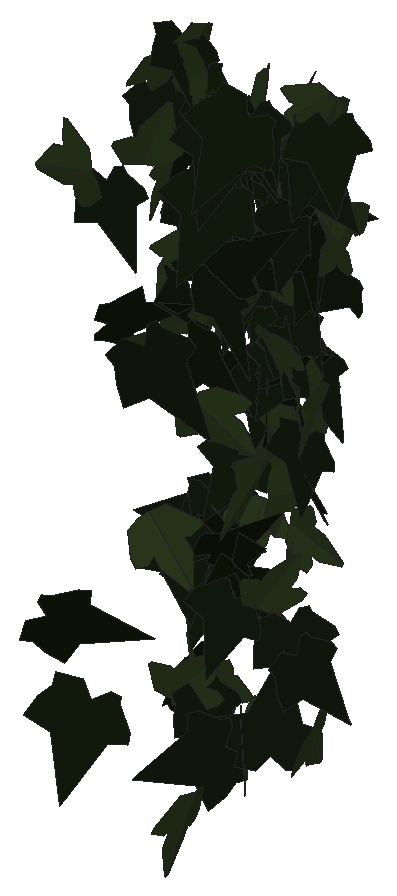
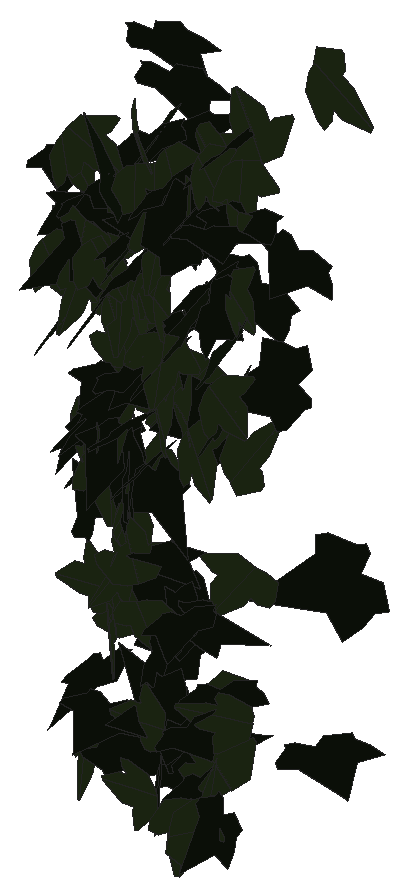
# SketchUp Ruby script. Lengths in inches.
U = 1.inch
M = Sketchup.active_model
def pt(a) = Geom::Point3d.new(a.map { |v| v * U })
def face(e, loops, mat)
  f = e.add_face(loops[0].map { |a| pt(a) })
  loops[1..].each { |l| e.add_face(l.map { |a| pt(a) }).erase! }
  f.material = f.back_material = mat if mat
  f
end
# faces: each face lists its corners as indices into pts; further lists are holes
def faces(e, pts, list, mat = nil) = list.each { |f| face(e, (f[0].is_a?(Array) ? f : [f]).map { |l| l.map { |i| pts[i] } }, mat) }
# xy, xz, yz: faces in a plane at the given z, y or x. An outline is a flat list of corners, or four numbers for a rectangle; further outlines are holes
def ring(l) = l.size == 4 ? [[l[0], l[1]], [l[2], l[1]], [l[2], l[3]], [l[0], l[3]]] : l.each_slice(2).to_a
def flat(e, list, mat, &to3) = list.each { |f| face(e, (f[0].is_a?(Array) ? f : [f]).map { |l| ring(l).map { |u, v| to3.(u, v) } }, mat) }
def xy(e, z, list, mat = nil) = flat(e, list, mat) { |x, y| [x, y, z] }
def xz(e, y, list, mat = nil) = flat(e, list, mat) { |x, z| [x, y, z] }
def yz(e, x, list, mat = nil) = flat(e, list, mat) { |y, z| [x, y, z] }
def lines(e, pts, list) = list.each { |a, b| e.add_line(pt(pts[a]), pt(pts[b])) }
# prism: a flat outline (further loops are holes) pulled along v
def prism(e, loops, v, mat = nil)
  f = face(e, loops, mat); d = Geom::Vector3d.new(v.map { |x| x * U })
  f.pushpull(f.normal.samedirection?(d) ? d.length : -d.length)
end
def box(e, o, s, mat = nil) = prism(e, [[o, [o[0] + s[0], o[1], o[2]], [o[0] + s[0], o[1] + s[1], o[2]], [o[0], o[1] + s[1], o[2]]]], [0, 0, s[2]], mat)
def at(x, y, z, deg = 0) = Geom::Transformation.translation(pt([x, y, z])) * Geom::Transformation.rotation(ORIGIN, Z_AXIS, deg.degrees)
def axes(o, x, y, z) = Geom::Transformation.new([*x, 0, *y, 0, *z, 0, *pt(o).to_a, 1])
def part(name) = M.definitions.add(name)
# library, detail: a bought-in or finely detailed component or shape, given as its bounding box
def library(name, o, s) = part(name).tap { |d| box(d.entities, o, s) }
def detail(e, o, s) = box(e.add_group.entities, o, s)
def put(e, d, t, mat = nil) = e.add_instance(d, t).tap { |i| i.material = mat if mat }
def group(e, t, mat = nil) = e.add_group.tap { |g| g.transformation = t; g.material = mat if mat }.entities
root = M.entities
M.materials.add("efeu1").color = [18, 25, 13]
M.materials.add("efeu2").color = [43, 57, 29]
c1 = part("ivyleaf_10")
p = [[0,0.5,-0.03],[-0.0625,2.02,-0.43],[-0.19,2.01,-0.46],[-0.54,1.05,-0.29],[-0.52,0.625,-0.18],[-0.83,0.76,-0.28],
  [-1.16,0.64,-0.33],[-1.15,0.33,-0.24],[-0.77,-0.39,0.02],[-0.3,-0.51,0.16],[0.04,-0.48,0.23],[-0.02,2.01,-0.4375],
  [-0.06,2.01,-0.43],[0.04,-0.49,0.23],[0.67,-0.49,0.14],[1.38,0.36,-0.2],[1.375,0.51,-0.24],[0.81,0.65,-0.19],
  [0.62,0.59,-0.15],[0.6,1.09,-0.28],[0.5,1.23,-0.31]]
faces(c1.entities,p,[[0,1,2,3,4,5,6,7,8,9,10],[11,12,0,13,14,15,16,17,18,19,20]],"efeu2")
c2 = part("ivyleaf_9")
p = [[1.54,2.16,1.25],[1.36,2.04,1.19],[-0.21,0.99,0.68],[-0.71,1.11,0.82],[-0.85,0.86,0.67],[-0.8,0.17,0.21],
  [-0.9,-0.01,0.1],[-0.67,-0.16,-0.02],[-0.08,-0.08,-0.05],[-0.03,-0.6,-0.4],[0.65,-0.88,-0.66],[0.83,-0.6,-0.49],
  [1.29,-0.42,-0.43],[1.8125,-0.07,-0.26],[1.21,0.44,0.15]]
faces(c2.entities,p,[[0,1,2,3,4,5,6,7,8,9,10,11,12,13,14]],"efeu1")
put(root,c1,axes([519.01,126.77,205.03],[-0.31987,0.03576,1.02162],[-1.02187,-0.04001,-0.31855],[0.02752,-1.06978,0.04607]))
put(root,c1,axes([521.88,127.9,184.67],[0.16584,-1.03656,0.26292],[0.06825,-0.25526,-1.04942],[1.06721,0.1774,0.02625]))
put(root,c2,axes([517.63,127,189.8],[0.13093,0.34043,-0.9819],[0.41581,0.88983,0.36395],[0.95243,-0.43528,-0.02391]))
put(root,c2,axes([520.05,128.35,198.8],[-0.14877,-0.30864,-1.04293],[0.82718,0.65139,-0.31076],[0.70622,-0.82797,0.14429]))
put(root,c2,axes([517.01,129.52,185.63],[-0.63548,-0.79383,-0.19057],[0.11492,0.15212,-1.01684],[0.80825,-0.64577,-0.00526]))
put(root,c2,axes([521.53,129.91,203.75],[-0.52245,-0.87618,0.11869],[-0.0636,-0.10026,-1.02012],[0.8819,-0.5263,-0.00326]))
put(root,c2,axes([522.52,129.74,206.55],[-0.92389,-0.45387,-0.15194],[0.13673,0.06627,-1.02935],[0.45868,-0.93395,0.0008]))
put(root,c2,axes([521.48,129.72,200.92],[0.47858,-0.90282,-0.01651],[-0.00454,0.01629,-1.02182],[0.90296,0.47859,0.00362]))
put(root,c2,axes([521.63,130.19,205.73],[-0.82447,-0.51633,-0.33937],[0.29967,0.16074,-0.97257],[0.54035,-0.87698,0.02155]))
put(root,c1,axes([518.93,129.84,204.1875],[-0.46617,-0.77023,0.19402],[0.10362,0.16408,0.90031],[-0.7875,0.47753,0.00361]))
put(root,c2,axes([521.22,129.75,200.97],[0.02313,-0.08298,1.0143],[1.00331,0.17177,-0.00883],[-0.17043,0.99992,0.08569]))
put(root,c2,axes([520.66,131,184.8],[-0.0399,-0.47857,-0.87325],[0.1005,-0.87143,0.47297],[-0.99071,-0.06912,0.08315]))
put(root,c1,axes([520.78,130.08,196.41],[-0.75552,-0.27252,-0.60479],[0.55997,0.22939,-0.80291],[0.35562,-0.94019,-0.0206]))
put(root,c1,axes([521.46,131.29,193.6],[0.19021,-0.33456,0.88892],[0.38201,-0.80307,-0.38399],[0.86959,0.42596,-0.02575]))
put(root,c2,axes([516.74,130.71,202],[-0.38724,-0.30191,-0.75298],[0.62895,0.41527,-0.48996],[0.51239,-0.7379,0.03234]))
put(root,c1,axes([518.38,130.89,191.24],[0.67878,0.4004,0.57075],[0.49981,0.27589,-0.78796],[-0.48606,0.84284,-0.01322]))
put(root,c2,axes([516.99,130.57,197.64],[0.43513,0.28551,0.7271],[0.5825,0.43596,-0.51978],[-0.52047,0.72661,0.02615]))
put(root,c1,axes([521.19,131.46,199.2],[0.23654,-0.91313,-0.24005],[0.05873,-0.23276,0.94327],[-0.94232,-0.24372,-0.00147]))
put(root,c2,axes([520.61,132.1,205],[0.46524,-0.7141,-0.10338],[-0.04716,0.09265,-0.85221],[0.72,0.46749,0.01098]))
put(root,c2,axes([519.81,132.57,188.63],[-0.23336,-0.81643,0.19969],[-0.03743,-0.19695,-0.84894],[0.83966,-0.23568,0.01765]))
put(root,c2,axes([520.83,132.21,204.93],[0.01502,-0.75793,-0.37824],[0.04097,0.3785,-0.75684],[0.84608,-0.00487,0.04336]))
put(root,c1,axes([518.375,132.03,185.42],[-0.64156,-0.45455,0.48942],[0.39772,0.28524,0.78626],[-0.53663,0.75483,-0.00239]))
put(root,c2,axes([518.7,132.1,196.88],[-0.01661,-0.01432,-0.94426],[0.8476,0.41621,-0.02122],[0.41642,-0.84775,0.00553]))
put(root,c2,axes([520.18,132.58,184.54],[0.08773,-0.14272,-0.8229],[0.78761,-0.26113,0.12926],[-0.27785,-0.78528,0.10657]))
put(root,c2,axes([521,132.64,200.29],[0.40363,-0.90769,0.0306],[-0.01224,0.02805,0.99339],[-0.90813,-0.40382,0.00021]))
put(root,c1,axes([520,132.31,204.36],[0.00735,-0.83915,0.07771],[0.00116,-0.07771,-0.83918],[0.84274,0.00742,0.00048]))
put(root,c1,axes([517.14,132.84,195.9375],[-0.13269,-0.35305,-0.84263],[-0.27619,-0.79613,0.37706],[-0.87086,0.30628,0.00881]))
put(root,c1,axes([521.41,132.15,189.47],[-0.34614,-0.67975,0.38224],[0.19274,0.33066,0.76256],[-0.75566,0.39571,0.01941]))
put(root,c2,axes([521.65,132.01,184.62],[-0.81437,-0.19451,0.51813],[0.5031,0.12392,0.83727],[-0.23061,0.95723,-0.00311]))
put(root,c2,axes([521.72,132.9375,201.58],[-0.10971,-0.79954,0.25874],[0.05016,-0.2667,-0.80287],[0.83887,-0.08862,0.08185]))
put(root,c2,axes([519.9,132.85,199.24],[-0.2366,-0.78834,0.02024],[-0.00511,-0.0196,-0.82308],[0.78858,-0.23665,0.00074]))
put(root,c2,axes([518.86,132.4375,185.26],[0.14733,-0.72504,-0.4325],[-0.07048,0.42694,-0.73973],[0.8413,0.16274,0.01377]))
put(root,c2,axes([518.31,132.75,201.31],[0.08268,-0.80664,-0.15809],[0.00292,0.15917,-0.81065],[0.82198,0.08057,0.01878]))
put(root,c2,axes([522.13,132.98,194.54],[-0.01234,-0.81617,0.10867],[0.0207,-0.10895,-0.81596],[0.82311,-0.0095,0.02215]))
put(root,c1,axes([518.64,132.41,205.61],[0.45137,-0.30497,-0.6524],[-0.50379,0.41648,-0.54324],[0.51462,0.6752,0.04041]))
put(root,c2,axes([519.3125,132.38,190.15],[0.50725,0.73315,-0.17413],[0.09541,0.14573,0.89151],[0.74748,-0.51613,0.00437]))
put(root,c2,axes([522.39,132.41,187.72],[0.27416,-0.5404,-0.6401],[-0.14338,0.6333,-0.59607],[0.82535,0.28952,0.10908]))
put(root,c2,axes([519.13,132.96,190.14],[0.10308,-0.20205,0.79884],[0.59706,-0.53653,-0.21274],[0.56789,0.60076,0.07867]))
put(root,c2,axes([521.96,133.23,192.98],[0.16199,-0.37225,0.7742],[0.36744,-0.68211,-0.40485],[0.77649,0.40044,0.03006]))
put(root,c1,axes([522.8,132.48,185.32],[0.08208,-0.72855,-0.48451],[-0.04713,0.48225,-0.73314],[0.87368,0.09446,0.00597]))
put(root,c2,axes([519.36,132.95,203.16],[-0.27153,-0.22066,-0.81665],[0.78986,0.24095,-0.32773],[0.30287,-0.82619,0.12253]))
put(root,c2,axes([518.49,133.35,203.74],[0.05889,-0.76881,0.33445],[0.05568,-0.33094,-0.77057],[0.83656,0.07615,0.02775]))
put(root,c1,axes([520.43,133.19,205.56],[0.5417,-0.4128,0.53936],[0.42723,-0.32923,-0.68106],[0.52801,0.68989,-0.00228]))
put(root,c2,axes([518.63,133.04,190.7],[-0.30926,-0.24955,-0.7248],[-0.564,-0.45524,0.39738],[-0.51915,0.64322,0.00005]))
put(root,c1,axes([516.95,133.27,201.7],[0.26054,-0.68935,0.42023],[0.17032,-0.3847,-0.73667],[0.78917,0.31061,0.02025]))
put(root,c2,axes([522.03,133.27,201.16],[-0.28354,-0.16781,-0.80142],[0.81859,-0.03867,-0.28152],[0.01876,-0.84922,0.17118]))
put(root,c1,axes([522.34,133.41,195.8],[0.2956,-0.62662,0.51847],[0.22332,-0.46791,-0.69284],[0.78205,0.37047,0.00187]))
put(root,c2,axes([517.5,133.22,205.96],[0.1942,-0.86612,-0.10074],[-0.00267,0.10262,-0.88741],[0.87196,0.19322,0.01972]))
put(root,c1,axes([520.3,133.12,184.66],[-0.16319,0.02788,-0.82667],[0.76294,-0.32042,-0.16141],[-0.31952,-0.77933,0.03679]))
put(root,c2,axes([517.41,133.59,197.23],[0.51341,-0.572,-0.38851],[0.24292,-0.30384,0.76836],[-0.64739,-0.56764,-0.01979]))
put(root,c1,axes([516.99,132.89,205.28],[-0.29687,-0.7823,-0.20791],[0.04851,0.20386,-0.83633],[0.808,-0.29967,-0.02617]))
put(root,c2,axes([519.0625,132.92,200.11],[0.25475,-0.64378,-0.46681],[0.03017,0.49765,-0.66985],[0.79464,0.18749,0.17509]))
put(root,c1,axes([520.125,133.49,200.42],[0.36037,-0.63469,0.58028],[0.34551,-0.4693,-0.72788],[0.78752,0.49634,0.0538]))
put(root,c1,axes([521.07,132.91,197.37],[-0.83559,0.17919,-0.02298],[0.02243,-0.00499,-0.85458],[-0.17926,-0.83589,0.00018]))
put(root,c2,axes([519.41,133.35,204.24],[0.06442,-0.83473,-0.10782],[-0.02085,0.10651,-0.83712],[0.84141,0.06655,-0.01249]))
put(root,c1,axes([520.64,133.03,203.88],[-0.25035,-0.89449,-0.17919],[0.04572,0.17328,-0.92886],[0.91112,-0.25448,-0.00263]))
put(root,c1,axes([518.93,132.875,204.1],[0.43706,-0.59727,-0.40094],[-0.0378,0.44943,-0.7107],[0.71837,0.38703,0.20654]))
put(root,c2,axes([516.82,133.01,204.17],[0.01524,-0.50716,-0.691],[0.23182,0.66779,-0.48501],[0.82519,-0.17824,0.14902]))
put(root,c1,axes([518.27,132.99,185.04],[-0.45876,0.62383,-0.26821],[-0.15675,0.21765,0.77435],[0.6607,0.48479,-0.00252]))
put(root,c1,axes([521.28,133.43,195.2],[-0.59796,0.25103,0.56603],[0.51544,-0.23423,0.6484],[0.34311,0.78935,0.01239]))
put(root,c2,axes([518.3,133.62,200.41],[0.37445,-0.72279,0.32065],[0.16106,-0.27762,-0.8139],[0.77415,0.40737,0.01424]))
put(root,c2,axes([519.26,133.93,189.87],[0.00676,-0.30434,-0.73503],[0.48942,-0.57791,0.24379],[-0.62719,-0.45424,0.18232]))
put(root,c1,axes([520.39,133.56,193.82],[0.00007,-0.7838,0.19781],[0.01809,-0.19776,-0.78361],[0.80818,0.00449,0.01752]))
put(root,c2,axes([519.43,133.78,192.8],[-0.60525,-0.52091,0.05023],[-0.04247,-0.02765,-0.79851],[0.5216,-0.6067,-0.00674]))
put(root,c1,axes([518.23,133.8,197.56],[0.0414,-0.15368,0.89806],[0.81371,-0.39818,-0.10565],[0.40987,0.80602,0.11904]))
put(root,c1,axes([521.34,133.42,194.85],[-0.70353,-0.48754,0.09608],[-0.07852,-0.05538,-0.85595],[0.49068,-0.7079,0.00079]))
put(root,c2,axes([521.56,134.04,199.625],[-0.00516,-0.68089,0.51153],[0.00471,-0.51155,-0.68088],[0.85162,-0.0013,0.00686]))
put(root,c2,axes([519.87,133.94,195.27],[-0.03297,-0.76151,0.28992],[0.05538,-0.29158,-0.75957],[0.81295,-0.01102,0.0635]))
put(root,c2,axes([522.49,133.65,204.55],[-0.25533,-0.75949,-0.34593],[0.15627,0.31185,-0.80001],[0.8198,-0.29599,0.04476]))
put(root,c1,axes([519.11,133.89,200.96],[0.24278,-0.5067,0.6357],[0.43119,-0.48216,-0.549],[0.68915,0.48018,0.11955]))
put(root,c2,axes([521.71,133.95,203.55],[-0.2227,-0.77074,0.15639],[-0.00639,-0.16076,-0.80138],[0.78642,-0.21957,0.03777]))
put(root,c2,axes([520.71,134.05,196.25],[-0.29328,-0.68596,0.31961],[-0.00346,-0.34156,-0.73623],[0.75676,-0.2674,0.1205]))
put(root,c1,axes([519.53,133.27,202.96],[-0.31978,-0.81806,-0.31942],[0.11037,0.2998,-0.87832],[0.87125,-0.33824,-0.00598]))
put(root,c1,axes([521.99,133.86,205.18],[-0.32421,-0.47892,0.60739],[-0.28369,-0.53907,-0.57648],[0.71959,-0.4283,0.04639]))
put(root,c2,axes([520.26,133.77,194.11],[-0.08204,0.39346,0.74912],[-0.0965,-0.75207,0.38445],[0.84064,-0.04793,0.11724]))
put(root,c1,axes([520.6,133.5,198.79],[-0.72321,-0.33241,0.3256],[0.30741,0.11041,0.79552],[-0.3493,0.7854,0.02598]))
put(root,c1,axes([522.78,133.34,201.11],[-0.71201,0.11709,0.42797],[-0.42877,0.02654,-0.72061],[-0.11411,-0.83031,0.03732]))
put(root,c1,axes([520.96,133.35,200.36],[-0.83385,0.14332,0.18917],[-0.18595,0.03485,-0.84607],[-0.14747,-0.85433,-0.00278]))
put(root,c2,axes([517.1,133.69,189.23],[-0.29533,-0.69787,-0.3868],[0.15918,0.35262,-0.75775],[0.78186,-0.3354,0.00816]))
put(root,c2,axes([519.14,133.97,198.89],[0.08514,-0.79086,0.19974],[-0.00289,-0.20112,-0.79508],[0.81569,0.08184,-0.02367]))
put(root,c1,axes([517.51,133.86,205.77],[0.05681,-0.77024,0.32291],[0.05172,-0.31979,-0.7719],[0.83359,0.07234,0.02589]))
put(root,c1,axes([521.47,133.56,191.03],[0.13233,-0.01742,0.84861],[0.84389,0.09486,-0.12965],[-0.09108,0.85361,0.03173]))
put(root,c2,axes([519.25,132.86,187.43],[-0.07008,0.57851,-0.58892],[-0.07644,0.58396,0.58273],[0.82199,0.10363,0.00398]))
put(root,c1,axes([521.5625,133.86,196.05],[-0.34481,0.324,-0.71447],[0.461,-0.54779,-0.4709],[-0.63476,-0.57384,0.04612]))
put(root,c2,axes([520.1875,133.65,202.64],[0.16457,-0.75663,-0.3218],[0.02874,0.33328,-0.76891],[0.82171,0.13988,0.09135]))
put(root,c1,axes([516.97,133.98,198.72],[-0.13053,-0.69259,0.43871],[-0.01143,-0.44266,-0.70222],[0.81977,-0.11645,0.06007]))
put(root,c2,axes([520.97,133.38,195.62],[0.46696,0.12425,-0.72216],[-0.71333,-0.11885,-0.4817],[-0.16766,0.85172,0.03813]))
put(root,c2,axes([516.75,134.11,200.15],[0.20166,-0.72001,0.34686],[0.10778,-0.32996,-0.7476],[0.7919,0.22826,0.01342]))
put(root,c1,axes([517.87,133.9,196.89],[0.03786,-0.88419,0.20304],[0.04706,-0.20103,-0.88421],[0.90598,0.04739,0.03744]))
put(root,c1,axes([520.22,134.18,193.75],[-0.15705,0.26463,0.78438],[0.40507,-0.6717,0.30772],[0.72194,0.43445,-0.00202]))
put(root,c2,axes([518.27,133.5625,203.24],[0.55611,-0.12227,0.71843],[0.70289,-0.14862,-0.56939],[0.19242,0.89627,0.00359]))
put(root,c1,axes([518.09,134.24,184.65],[0.08115,0.10556,-0.80531],[-0.42051,-0.68695,-0.13241],[-0.69487,0.42804,-0.01391]))
put(root,c2,axes([520.85,133.62,203.76],[-0.12543,0.72562,0.44241],[0.02695,-0.44359,0.73518],[0.84943,0.12122,0.04201]))
put(root,c1,axes([521.18,134.05,201.87],[-0.474,-0.58104,0.39007],[-0.0931,-0.41458,-0.73069],[0.69361,-0.45272,0.16849]))
put(root,c2,axes([521.6875,133.72,202.99],[-0.01895,-0.43085,-0.7109],[0.52556,0.54472,-0.34415],[0.64405,-0.45718,0.25991]))
put(root,c2,axes([518.32,133.89,191.25],[-0.14095,-0.68707,-0.3531],[0.09434,0.34093,-0.70106],[0.76671,-0.16826,0.02135]))
put(root,c1,axes([519.72,133.87,190.96],[0.73617,0.27254,-0.1564],[-0.14559,-0.0572,-0.78499],[-0.27847,0.75042,-0.00303]))
put(root,c1,axes([522.16,134.1,204.9],[-0.10694,-0.75394,0.33237],[-0.00437,-0.33464,-0.76049],[0.82394,-0.09963,0.0391]))
put(root,c1,axes([518.26,133.75,184.92],[-0.83282,-0.24757,-0.02247],[0.02154,0.0064,-0.86884],[0.24765,-0.8331,0]))
put(root,c2,axes([519.91,134.3125,201.94],[0.01341,-0.80973,0.16957],[0.00682,-0.16948,-0.80983],[0.82726,0.01452,0.00392]))
put(root,c2,axes([519.96,134.09,202.6],[0.4197,-0.79627,0.01693],[0.00762,-0.01512,-0.9001],[0.79641,0.41977,-0.00031]))
put(root,c1,axes([521.68,133.93,202.45],[0.83809,0.02697,0.36476],[0.36465,0.0092,-0.83852],[-0.0284,0.91398,-0.00232]))
put(root,c2,axes([518.83,134,188.02],[-0.08594,-0.06716,0.83269],[0.67213,-0.50267,0.02882],[0.49611,0.66939,0.10519]))
put(root,c2,axes([521.09,133.32,196.08],[0.26762,0.81005,0.16758],[0.0622,0.15592,-0.85305],[-0.82486,0.27457,-0.00996]))
put(root,c2,axes([519.29,133.81,195.38],[0.30892,0.16969,-0.77235],[-0.69342,-0.34046,-0.35215],[-0.38012,0.75898,0.01472]))
put(root,c2,axes([520.88,133.93,187.57],[-0.2443,-0.53499,-0.67189],[0.40597,0.54365,-0.58049],[0.75686,-0.46429,0.09449]))
put(root,c1,axes([519.94,134.01,192.3125],[-0.47632,-0.68564,0.09174],[0.07039,0.06276,0.83457],[-0.68816,0.48099,0.02187]))
put(root,c1,axes([520.95,133.75,190.23],[0.42172,-0.55874,-0.39346],[-0.12849,0.38927,-0.69051],[0.67118,0.42558,0.11503]))
put(root,c2,axes([517.36,133.35,185],[-0.12877,0.18977,-0.77358],[-0.44458,0.63308,0.22931],[0.6609,0.46284,0.00353]))
put(root,c2,axes([517.05,134.375,204.18],[-0.49599,-0.62896,-0.24306],[0.27783,0.08431,-0.7851],[0.6144,-0.54588,0.1588]))
put(root,c2,axes([520.01,134.44,198.68],[-0.36925,-0.70041,0.04303],[-0.01276,-0.04191,-0.79174],[0.70162,-0.36938,0.00825]))
put(root,c2,axes([517.61,134.45,188.24],[-0.35372,-0.80074,-0.03054],[0.00911,0.02937,-0.87538],[0.80127,-0.35382,-0.00353]))
put(root,c1,axes([522.68,134.35,201.51],[-0.13915,-0.74986,0.33585],[0.04011,-0.34643,-0.75686],[0.82066,-0.11022,0.09394]))
put(root,c2,axes([521.4375,134.08,196.45],[0.24093,-0.76841,-0.33949],[-0.04262,0.34154,-0.80329],[0.83898,0.23801,0.05669]))
put(root,c2,axes([522.3,134.71,199.24],[-0.15788,-0.49117,0.63866],[0.00883,-0.65182,-0.49911],[0.80564,-0.08911,0.13063]))
put(root,c2,axes([521.66,133.43,201.72],[0.07646,0.16267,-0.84513],[-0.05843,0.84749,0.15784],[0.85866,0.04319,0.086]))
put(root,c1,axes([522,133.7,200.82],[-0.14715,-0.67314,-0.56509],[0.10244,0.55591,-0.68889],[0.8729,-0.17872,-0.01441]))
put(root,c2,axes([520.81,133.81,197.32],[0.28375,-0.47267,-0.59942],[-0.08181,0.61698,-0.52524],[0.75896,0.24321,0.16749]))
put(root,c2,axes([520.45,134.1,198.24],[-0.18836,-0.53119,-0.68217],[0.41107,0.5592,-0.54893],[0.76062,-0.43375,0.12773]))
put(root,c1,axes([518.94,134.04,199.62],[-0.78344,-0.3182,-0.0267],[0.02461,0.01037,-0.8456],[0.31837,-0.78383,-0.00035]))
put(root,c1,axes([520.59,133.54,191.96],[0.08172,-0.302,-0.79484],[0.17649,0.78714,-0.28093],[0.83176,-0.13735,0.1377]))
put(root,c2,axes([516.75,134.54,202.02],[-0.20776,0.21973,-0.78211],[0.55835,-0.54777,-0.30221],[-0.5901,-0.59566,-0.01059]))
put(root,c1,axes([519.09,134.13,187.65],[0.04996,-0.01483,0.82486],[0.81696,0.11589,-0.0474],[-0.11481,0.8182,0.02167]))
put(root,c1,axes([516.42,133.86,188.6],[0.16846,-0.03138,-0.82619],[0.79335,0.24348,0.15252],[0.23273,-0.80727,0.07812]))
put(root,c1,axes([518.4,134.53,197.4375],[-0.20785,0.02509,0.85234],[0.75412,-0.40407,0.1958],[0.398,0.77872,0.07413]))
